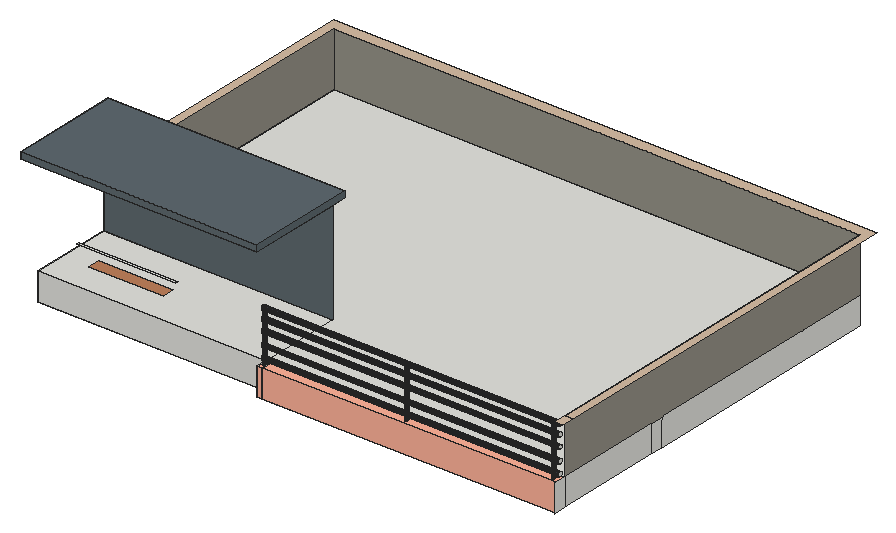
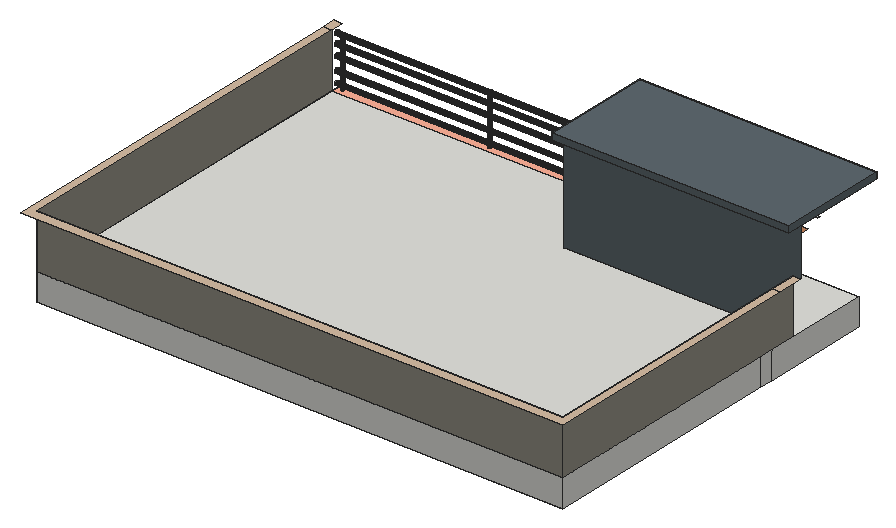
# SketchUp Ruby script. Lengths in inches.
U = 1.inch
M = Sketchup.active_model
def pt(a) = Geom::Point3d.new(a.map { |v| v * U })
def face(e, loops, mat)
  f = e.add_face(loops[0].map { |a| pt(a) })
  loops[1..].each { |l| e.add_face(l.map { |a| pt(a) }).erase! }
  f.material = f.back_material = mat if mat
  f
end
# faces: each face lists its corners as indices into pts; further lists are holes
def faces(e, pts, list, mat = nil) = list.each { |f| face(e, (f[0].is_a?(Array) ? f : [f]).map { |l| l.map { |i| pts[i] } }, mat) }
# xy, xz, yz: faces in a plane at the given z, y or x. An outline is a flat list of corners, or four numbers for a rectangle; further outlines are holes
def ring(l) = l.size == 4 ? [[l[0], l[1]], [l[2], l[1]], [l[2], l[3]], [l[0], l[3]]] : l.each_slice(2).to_a
def flat(e, list, mat, &to3) = list.each { |f| face(e, (f[0].is_a?(Array) ? f : [f]).map { |l| ring(l).map { |u, v| to3.(u, v) } }, mat) }
def xy(e, z, list, mat = nil) = flat(e, list, mat) { |x, y| [x, y, z] }
def xz(e, y, list, mat = nil) = flat(e, list, mat) { |x, z| [x, y, z] }
def yz(e, x, list, mat = nil) = flat(e, list, mat) { |y, z| [x, y, z] }
def lines(e, pts, list) = list.each { |a, b| e.add_line(pt(pts[a]), pt(pts[b])) }
# prism: a flat outline (further loops are holes) pulled along v
def prism(e, loops, v, mat = nil)
  f = face(e, loops, mat); d = Geom::Vector3d.new(v.map { |x| x * U })
  f.pushpull(f.normal.samedirection?(d) ? d.length : -d.length)
end
def box(e, o, s, mat = nil) = prism(e, [[o, [o[0] + s[0], o[1], o[2]], [o[0] + s[0], o[1] + s[1], o[2]], [o[0], o[1] + s[1], o[2]]]], [0, 0, s[2]], mat)
def at(x, y, z, deg = 0) = Geom::Transformation.translation(pt([x, y, z])) * Geom::Transformation.rotation(ORIGIN, Z_AXIS, deg.degrees)
def axes(o, x, y, z) = Geom::Transformation.new([*x, 0, *y, 0, *z, 0, *pt(o).to_a, 1])
def part(name) = M.definitions.add(name)
# library, detail: a bought-in or finely detailed component or shape, given as its bounding box
def library(name, o, s) = part(name).tap { |d| box(d.entities, o, s) }
def detail(e, o, s) = box(e.add_group.entities, o, s)
def put(e, d, t, mat = nil) = e.add_instance(d, t).tap { |i| i.material = mat if mat }
def group(e, t, mat = nil) = e.add_group.tap { |g| g.transformation = t; g.material = mat if mat }.entities
root = M.entities
M.materials.add("[Color B02]").color = [255, 178, 153]
M.materials.add("[Formica Graystone]").color = [149, 146, 135]
M.materials.add("[Formica Laminate Dark]").color = [50, 53, 60]
M.materials.add("[Formica Laminate Light]").color = [213, 189, 164]
M.materials.add("[Formica Speckled Grey]").color = [94, 105, 111]
M.materials.add("[Mirror 02]").color = [229, 229, 229]
M.materials.add("[Translucent Glass Gray]").color = [128, 128, 128]
M.materials["[Translucent Glass Gray]"].alpha = 0.5
M.materials.add("[Wood Veneer 02]").color = [190, 128, 91]
xy(root,233.31,[[241.28,125.15,282.74,137.68]])
xy(root,236.52,[[343.11,125.15,391.96,137.68]])
xy(root,253.98,[[7.28,125.15,478.18,137.68],[7.28,137.68,478.18,359.0625]])
xy(root,253.98,[[211.9,17.0625,211.86,27.5,7.28,27.5,7.28,125.15,478.18,125.15,478.18,28.71,478.21,17.0625,478.18,17.0625,478.17,18.28,216.21,17.09,216.18,27.52,216.17,27.53,216.21,17.09,211.9375,17.0625]],"[Color B02]")
xy(root,278.46,[[216.21,17.09,216.18,27.52,216.17,27.52],[214.34,20.96,214.03,21.01,213.73,21.16,213.48,21.4,213.29,21.71,213.17,22.07,213.13,22.46,213.17,22.85,213.29,23.21,213.48,23.52,213.73,23.76,214.03,23.91,214.34,23.96,214.66,23.91,214.95,23.76,215.2,23.52,215.39,23.21,215.51,22.85,215.55,22.46,215.51,22.07,215.39,21.71,215.2,21.4,214.95,21.16,214.66,21.01],[341.47,20.96,341.16,21.01,340.86,21.16,340.61,21.4,340.42,21.71,340.3,22.07,340.26,22.46,340.3,22.85,340.42,23.21,340.61,23.52,340.86,23.76,341.16,23.91,341.47,23.96,341.79,23.91,342.08,23.76,342.33,23.52,342.52,23.21,342.64,22.85,342.68,22.46,342.64,22.07,342.52,21.71,342.33,21.4,342.08,21.16,341.79,21.01],[473.1,20.96,472.79,21.01,472.49,21.16,472.24,21.4,472.05,21.71,471.93,22.07,471.89,22.46,471.93,22.85,472.05,23.21,472.24,23.52,472.49,23.76,472.79,23.91,473.1,23.96,473.42,23.91,473.71,23.76,473.96,23.52,474.15,23.21,474.27,22.85,474.32,22.46,474.27,22.07,474.15,21.71,473.96,21.4,473.71,21.16,473.42,21.01],[211.9,27.5,216.17,27.52,216.17,27.53,216.18,27.52,478.18,28.71,478.18,359.0625,7.28,359.0625,7.28,101.5625,211.9,101.5625],
  [7.28,27.5,211.9,101.5625],[216.17,27.52,216.18,27.52,216.17,27.53]])
xy(root,278.46,[[[211.9,17.0625,211.9375,17.0625,216.21,17.09,216.17,27.52,211.9,27.5,211.86,27.5],[214.34,20.96,214.03,21.01,213.73,21.16,213.48,21.4,213.29,21.71,213.17,22.07,213.13,22.46,213.17,22.85,213.29,23.21,213.48,23.52,213.73,23.76,214.03,23.91,214.34,23.96,214.66,23.91,214.95,23.76,215.2,23.52,215.39,23.21,215.51,22.85,215.55,22.46,215.51,22.07,215.39,21.71,215.2,21.4,214.95,21.16,214.66,21.01]],[[478.18,17.0625,478.21,17.0625,478.18,28.71,216.18,27.52,216.21,17.09,478.17,18.28],[473.1,20.96,472.79,21.01,472.49,21.16,472.24,21.4,472.05,21.71,471.93,22.07,471.89,22.46,471.93,22.85,472.05,23.21,472.24,23.52,472.49,23.76,472.79,23.91,473.1,23.96,473.42,23.91,473.71,23.76,473.96,23.52,474.15,23.21,474.27,22.85,474.32,22.46,474.27,22.07,474.15,21.71,473.96,21.4,473.71,21.16,473.42,21.01],[341.47,20.96,341.16,21.01,340.86,21.16,340.61,21.4,340.42,21.71,340.3,22.07,340.26,22.46,340.3,22.85,340.42,23.21,340.61,23.52,340.86,23.76,341.16,23.91,341.47,23.96,341.79,23.91,342.08,23.76,342.33,23.52,342.52,23.21,342.64,22.85,342.68,22.46,342.64,22.07,342.52,21.71,342.33,21.4,342.08,21.16,341.79,21.01]]],"[Color B02]")
xy(root,306.94,[[63.47,14.6875,129.94,25.8125]],"[Wood Veneer 02]")
xy(root,321.27,[[52.1,14.6875,141.31,17.0625]])
xy(root,323.28,[[473.1,20.96,473.42,21.01,473.71,21.16,473.96,21.4,474.15,21.71,474.27,22.07,474.32,22.46,474.27,22.85,474.15,23.21,473.96,23.52,473.71,23.76,473.42,23.91,473.1,23.96,472.79,23.91,472.49,23.76,472.24,23.52,472.05,23.21,471.93,22.85,471.89,22.46,471.93,22.07,472.05,21.71,472.24,21.4,472.49,21.16,472.79,21.01]])
xy(root,323.89,[[341.47,20.96,341.79,21.01,342.08,21.16,342.33,21.4,342.52,21.71,342.64,22.07,342.66,22.1875,340.29,22.1875,340.3,22.07,340.42,21.71,340.61,21.4,340.86,21.16,341.16,21.01],[340.29,22.1875,342.66,22.1875,342.68,22.46,342.64,22.85,342.52,23.21,342.33,23.52,342.08,23.76,341.79,23.91,341.47,23.96,341.16,23.91,340.86,23.76,340.61,23.52,340.42,23.21,340.3,22.85,340.26,22.46]])
xy(root,324.26,[[214.34,20.96,214.66,21.01,214.95,21.16,215.2,21.4,215.39,21.71,215.51,22.07,215.55,22.46,215.55,22.47,213.13,22.47,213.13,22.46,213.17,22.07,213.29,21.71,213.48,21.4,213.73,21.16,214.03,21.01],[213.13,22.47,215.55,22.47,215.51,22.85,215.39,23.21,215.2,23.52,214.95,23.76,214.66,23.91,214.34,23.96,214.03,23.91,213.73,23.76,213.48,23.52,213.29,23.21,213.17,22.85]])
xy(root,327.42,[[478.18,17.0625,485.46,28.71],[478.18,28.71,485.46,28.71,485.46,368.0625,0,368.0625,0,125.15,7.28,125.15,7.28,359.0625,478.18,359.0625],[0,101.5625,7.28,125.15]],"[Formica Laminate Light]")
xy(root,370.36,[[0,17.0625,211.9,101.5625],[0,101.5625,211.9,115.3125]])
xy(root,376.1875,[[0,17.0625,211.9,115.3125]],"[Formica Speckled Grey]")
xz(root,17.0625,[[211.9,253.98,211.9375,278.46],[478.18,253.98,478.21,278.46]])
xz(root,17.0625,[[0,370.36,211.9,376.1875]],"[Formica Speckled Grey]")
xz(root,27.5,[[7.28,253.98,211.86,278.46],[211.86,253.98,211.9,278.46]])
xz(root,101.5625,[[7.28,278.46,7.28,327.42,0,327.42,0,370.36,211.9,370.36,211.9,278.46]],"[Formica Speckled Grey]")
xz(root,115.3125,[[0,370.36,211.9,376.1875]],"[Formica Speckled Grey]")
xz(root,125.15,[[245.46,221.85,260.12,228.03],[263.78,221.85,278.56,228.03]],"[Mirror 02]")
xz(root,125.15,[[346.84,218.58,365.15,225.02],[369.6875,218.58,388.23,225.02],[346.84,225.02,365.15,231.81],[369.6875,225.02,388.23,231.81]],"[Translucent Glass Gray]")
xz(root,359.0625,[[7.28,253.98,478.18,278.46]])
xz(root,359.0625,[[7.28,278.46,478.18,327.42]],"[Formica Graystone]")
yz(root,0,[[17.0625,370.36,115.3125,376.1875]],"[Formica Speckled Grey]")
yz(root,7.28,[[27.5,253.98,125.15,278.46],[125.15,253.98,137.68,278.46],[137.68,253.98,359.0625,278.46]])
yz(root,7.28,[[101.5625,278.46,359.0625,327.42]],"[Formica Graystone]")
yz(root,211.9,[[17.0625,370.36,115.3125,376.1875]],"[Formica Speckled Grey]")
yz(root,478.18,[[28.71,253.98,125.15,278.46],[125.15,253.98,137.68,278.46],[137.68,253.98,359.0625,278.46],[23.7,280.86,24.16,280.92,24.58,281.1,24.94,281.38,25.22,281.75,25.4,282.18,25.45,282.64,25.4,283.11,25.22,283.54,24.94,283.91,24.58,284.19,24.16,284.37,23.7,284.43,23.25,284.37,22.83,284.19,22.47,283.91,22.1875,283.54,22.01,283.11,21.95,282.64,22.01,282.18,22.1875,281.75,22.47,281.38,22.83,281.1,23.25,280.92],[23.7,291,24.16,291.06,24.58,291.23,24.94,291.52,25.22,291.89,25.4,292.32,25.45,292.78,25.4,293.24,25.22,293.67,24.94,294.04,24.58,294.33,24.16,294.5,23.7,294.57,23.25,294.5,22.83,294.33,22.47,294.04,22.1875,293.67,22.01,293.24,21.95,292.78,22.01,292.32,22.1875,291.89,22.47,291.52,22.83,291.23,23.25,291.06],
  [23.7,302.73,24.16,302.79,24.58,302.96,24.94,303.25,25.22,303.62,25.4,304.05,25.45,304.51,25.4,304.97,25.22,305.4,24.94,305.77,24.58,306.06,24.16,306.23,23.7,306.3,23.25,306.23,22.83,306.06,22.47,305.77,22.1875,305.4,22.01,304.97,21.95,304.51,22.01,304.05,22.1875,303.62,22.47,303.25,22.83,302.96,23.25,302.79],[23.7,312.48,24.16,312.54,24.58,312.72,24.94,313,25.22,313.37,25.4,313.8,25.45,314.26,25.4,314.73,25.22,315.16,24.94,315.53,24.58,315.81,24.16,315.99,23.7,316.05,23.25,315.99,22.83,315.81,22.47,315.53,22.1875,315.16,22.01,314.73,21.95,314.26,22.01,313.8,22.1875,313.37,22.47,313,22.83,312.72,23.25,312.54],[23.7,321.21,24.16,321.27,24.58,321.45,24.94,321.74,25.22,322.11,25.4,322.54,25.45,323,25.4,323.46,25.22,323.89,24.94,324.26,24.58,324.54,24.16,324.72,23.7,324.78,23.25,324.72,22.83,324.54,22.47,324.26,22.1875,323.89,22.01,323.46,21.95,323,22.01,322.54,22.1875,322.11,22.47,321.74,22.83,321.45,23.25,321.27]])
yz(root,478.18,[[28.71,278.46,359.0625,327.42]],"[Formica Graystone]")
p = [[211.9375,17.0625,253.98],[216.21,17.09,253.98],[216.21,17.09,278.46],[211.9375,17.0625,278.46],[211.86,27.5,278.46],[211.86,27.5,253.98],
  [211.9,17.0625,253.98],[211.9,17.0625,278.46],[216.18,27.52,253.98],[216.18,27.52,278.46],[478.17,18.28,253.98],[478.17,18.28,278.46],
  [216.17,27.53,253.98],[216.17,27.53,278.46],[216.17,27.52,278.46],[478.18,28.71,253.98],[478.18,28.71,278.46],[478.21,17.0625,278.46],
  [478.21,17.0625,253.98],[478.18,17.0625,253.98],[478.18,17.0625,278.46],[213.73,21.16,278.46],[214.03,21.01,278.46],[214.03,21.01,324.26],
  [213.73,21.16,324.26],[214.34,20.96,278.46],[214.34,20.96,324.26],[214.66,21.01,278.46],[214.66,21.01,324.26],[214.95,21.16,278.46],
  [214.95,21.16,324.26],[340.86,21.16,278.46],[341.16,21.01,278.46],[341.16,21.01,323.89],[340.86,21.16,323.89],[341.47,20.96,278.46],
  [341.47,20.96,323.89],[341.79,21.01,278.46],[341.79,21.01,323.89],[342.08,21.16,278.46],[342.08,21.16,323.89],[472.49,21.16,278.46],
  [472.79,21.01,278.46],[472.79,21.01,323.28],[472.49,21.16,323.28],[473.1,20.96,278.46],[473.1,20.96,323.28],[473.42,21.01,278.46],
  [473.42,21.01,323.28],[473.71,21.16,278.46],[473.71,21.16,323.28],[213.48,21.4,278.46],[213.48,21.4,324.26],[215.2,21.4,278.46],
  [215.2,21.4,324.26],[340.61,21.4,278.46],[340.61,21.4,323.89],[342.33,21.4,278.46],[342.33,21.4,323.89],[472.24,21.4,278.46],
  [472.24,21.4,323.28],[473.96,21.4,278.46],[473.96,21.4,323.28],[213.29,21.71,278.46],[213.29,21.71,324.26],[215.39,21.71,278.46],
  [215.39,21.71,324.26],[340.42,21.71,278.46],[340.42,21.71,323.89],[342.52,21.71,278.46],[342.52,21.71,323.89],[472.05,21.71,278.46],
  [472.05,21.71,323.28],[474.15,21.71,278.46],[474.15,21.71,323.28],[213.17,22.07,278.46],[213.17,22.07,324.26],[215.51,22.07,278.46],
  [215.51,22.07,324.26],[340.3,22.07,278.46],[340.3,22.07,323.89],[342.64,22.07,278.46],[342.64,22.07,323.89],[471.93,22.07,278.46],
  [471.93,22.07,323.28],[474.27,22.07,278.46],[474.27,22.07,323.28],[213.13,22.46,278.46],[213.13,22.46,324.26],[215.55,22.46,278.46],
  [215.55,22.46,324.26],[340.26,22.46,278.46],[340.29,22.1875,323.89],[340.26,22.46,323.89],[342.68,22.46,278.46],[342.68,22.46,323.89],
  [342.66,22.1875,323.89],[471.89,22.46,278.46],[471.89,22.46,323.28],[474.32,22.46,278.46],[474.32,22.46,323.28],[213.17,22.85,278.46],
  [213.13,22.47,324.26],[213.17,22.85,324.26],[215.51,22.85,278.46],[215.51,22.85,324.26],[215.55,22.47,324.26],[340.3,22.85,278.46],
  [340.3,22.85,323.89],[342.64,22.85,278.46],[342.64,22.85,323.89],[471.93,22.85,278.46],[471.93,22.85,323.28],[474.27,22.85,278.46],
  [474.27,22.85,323.28],[213.29,23.21,278.46],[213.29,23.21,324.26],[215.39,23.21,278.46],[215.39,23.21,324.26],[340.42,23.21,278.46],
  [340.42,23.21,323.89],[342.52,23.21,278.46],[342.52,23.21,323.89],[472.05,23.21,278.46],[472.05,23.21,323.28],[474.15,23.21,278.46],
  [474.15,23.21,323.28],[213.48,23.52,278.46],[213.48,23.52,324.26],[215.2,23.52,278.46],[215.2,23.52,324.26],[340.61,23.52,278.46],
  [340.61,23.52,323.89],[342.33,23.52,278.46],[342.33,23.52,323.89],[472.24,23.52,278.46],[472.24,23.52,323.28],[473.96,23.52,278.46],
  [473.96,23.52,323.28],[213.73,23.76,278.46],[213.73,23.76,324.26],[214.95,23.76,278.46],[214.95,23.76,324.26],[340.86,23.76,278.46],
  [340.86,23.76,323.89],[342.08,23.76,278.46],[342.08,23.76,323.89],[472.49,23.76,278.46],[472.49,23.76,323.28],[473.71,23.76,278.46],
  [473.71,23.76,323.28],[214.03,23.91,278.46],[214.03,23.91,324.26],[214.66,23.91,278.46],[214.66,23.91,324.26],[341.16,23.91,278.46],
  [341.16,23.91,323.89],[341.79,23.91,278.46],[341.79,23.91,323.89],[472.79,23.91,278.46],[472.79,23.91,323.28],[473.42,23.91,278.46],
  [473.42,23.91,323.28],[214.34,23.96,278.46],[214.34,23.96,324.26],[341.47,23.96,278.46],[341.47,23.96,323.89],[473.1,23.96,278.46],
  [473.1,23.96,323.28],[478.18,23.25,280.92],[478.18,22.83,281.1],[211.9,22.83,281.1],[211.9,23.25,280.92],[478.18,23.7,280.86],
  [211.9,23.7,280.86],[478.18,24.16,280.92],[211.9,24.16,280.92],[478.18,24.58,281.1],[211.9,24.58,281.1],[478.18,22.47,281.38],
  [211.9,22.47,281.38],[478.18,24.94,281.38],[211.9,24.94,281.38],[478.18,22.1875,281.75],[211.9,22.1875,281.75],[478.18,25.22,281.75],
  [211.9,25.22,281.75],[478.18,22.01,282.18],[211.9,22.01,282.18],[478.18,25.4,282.18],[211.9,25.4,282.18],[478.18,21.95,282.64],
  [211.9,21.95,282.64],[478.18,25.45,282.64],[211.9,25.45,282.64],[478.18,22.01,283.11],[211.9,22.01,283.11],[478.18,25.4,283.11],
  [211.9,25.4,283.11],[478.18,22.1875,283.54],[211.9,22.1875,283.54],[478.18,25.22,283.54],[211.9,25.22,283.54],[478.18,22.47,283.91],
  [211.9,22.47,283.91],[478.18,24.94,283.91],[211.9,24.94,283.91],[478.18,22.83,284.19],[211.9,22.83,284.19],[478.18,24.58,284.19],
  [211.9,24.58,284.19],[478.18,23.25,284.37],[211.9,23.25,284.37],[478.18,24.16,284.37],[211.9,24.16,284.37],[478.18,23.7,284.43],
  [211.9,23.7,284.43],[478.18,23.7,291],[478.18,23.25,291.06],[211.9,23.25,291.06],[211.9,23.7,291],[478.18,24.16,291.06],
  [211.9,24.16,291.06],[478.18,22.83,291.23],[211.9,22.83,291.23],[478.18,24.58,291.23],[211.9,24.58,291.23],[478.18,22.47,291.52],
  [211.9,22.47,291.52],[478.18,24.94,291.52],[211.9,24.94,291.52],[478.18,22.1875,291.89],[211.9,22.1875,291.89],[478.18,25.22,291.89],
  [211.9,25.22,291.89],[478.18,22.01,292.32],[211.9,22.01,292.32],[478.18,25.4,292.32],[211.9,25.4,292.32],[478.18,21.95,292.78],
  [211.9,21.95,292.78],[478.18,25.45,292.78],[211.9,25.45,292.78],[478.18,22.01,293.24],[211.9,22.01,293.24],[478.18,25.4,293.24],
  [211.9,25.4,293.24],[478.18,22.1875,293.67],[211.9,22.1875,293.67],[478.18,25.22,293.67],[211.9,25.22,293.67],[478.18,22.47,294.04],
  [211.9,22.47,294.04],[478.18,24.94,294.04],[211.9,24.94,294.04],[478.18,22.83,294.33],[211.9,22.83,294.33],[478.18,24.58,294.33],
  [211.9,24.58,294.33],[478.18,23.25,294.5],[211.9,23.25,294.5],[478.18,24.16,294.5],[211.9,24.16,294.5],[478.18,23.7,294.57],
  [211.9,23.7,294.57],[478.18,23.7,302.73],[478.18,23.25,302.79],[211.9,23.25,302.79],[211.9,23.7,302.73],[478.18,24.16,302.79],
  [211.9,24.16,302.79],[478.18,22.83,302.96],[211.9,22.83,302.96],[478.18,24.58,302.96],[211.9,24.58,302.96],[478.18,22.47,303.25],
  [211.9,22.47,303.25],[478.18,24.94,303.25],[211.9,24.94,303.25],[478.18,22.1875,303.62],[211.9,22.1875,303.62],[478.18,25.22,303.62],
  [211.9,25.22,303.62],[478.18,22.01,304.05],[211.9,22.01,304.05],[478.18,25.4,304.05],[211.9,25.4,304.05],[478.18,21.95,304.51],
  [211.9,21.95,304.51],[478.18,25.45,304.51],[211.9,25.45,304.51],[478.18,22.01,304.97],[211.9,22.01,304.97],[478.18,25.4,304.97],
  [211.9,25.4,304.97],[478.18,22.1875,305.4],[211.9,22.1875,305.4],[478.18,25.22,305.4],[211.9,25.22,305.4],[478.18,22.47,305.77],
  [211.9,22.47,305.77],[478.18,24.94,305.77],[211.9,24.94,305.77],[478.18,22.83,306.06],[211.9,22.83,306.06],[478.18,24.58,306.06],
  [211.9,24.58,306.06],[478.18,23.25,306.23],[211.9,23.25,306.23],[478.18,24.16,306.23],[211.9,24.16,306.23],[478.18,23.7,306.3],
  [211.9,23.7,306.3],[478.18,23.25,312.54],[478.18,22.83,312.72],[211.9,22.83,312.72],[211.9,23.25,312.54],[478.18,23.7,312.48],
  [211.9,23.7,312.48],[478.18,24.16,312.54],[211.9,24.16,312.54],[478.18,24.58,312.72],[211.9,24.58,312.72],[478.18,22.47,313],
  [211.9,22.47,313],[478.18,24.94,313],[211.9,24.94,313],[478.18,22.1875,313.37],[211.9,22.1875,313.37],[478.18,25.22,313.37],
  [211.9,25.22,313.37],[478.18,22.01,313.8],[211.9,22.01,313.8],[478.18,25.4,313.8],[211.9,25.4,313.8],[478.18,21.95,314.26],
  [211.9,21.95,314.26],[478.18,25.45,314.26],[211.9,25.45,314.26],[478.18,22.01,314.73],[211.9,22.01,314.73],[478.18,25.4,314.73],
  [211.9,25.4,314.73],[478.18,22.1875,315.16],[211.9,22.1875,315.16],[478.18,25.22,315.16],[211.9,25.22,315.16],[478.18,22.47,315.53],
  [211.9,22.47,315.53],[478.18,24.94,315.53],[211.9,24.94,315.53],[478.18,22.83,315.81],[211.9,22.83,315.81],[478.18,24.58,315.81],
  [211.9,24.58,315.81],[478.18,23.25,315.99],[211.9,23.25,315.99],[478.18,24.16,315.99],[211.9,24.16,315.99],[478.18,23.7,316.05],
  [211.9,23.7,316.05],[478.18,23.7,321.21],[478.18,23.25,321.27],[211.9,23.25,321.27],[211.9,23.7,321.21],[478.18,24.16,321.27],
  [211.9,24.16,321.27],[478.18,22.83,321.45],[211.9,22.83,321.45],[478.18,24.58,321.45],[211.9,24.58,321.45],[478.18,22.47,321.74],
  [211.9,22.47,321.74],[478.18,24.94,321.74],[211.9,24.94,321.74],[478.18,22.1875,322.11],[211.9,22.1875,322.11],[478.18,25.22,322.11],
  [211.9,25.22,322.11],[478.18,22.01,322.54],[211.9,22.01,322.54],[478.18,25.4,322.54],[211.9,25.4,322.54],[478.18,21.95,323],
  [211.9,21.95,323],[478.18,25.45,323],[211.9,25.45,323],[478.18,22.01,323.46],[211.9,22.01,323.46],[478.18,25.4,323.46],
  [211.9,25.4,323.46],[478.18,22.1875,323.89],[211.9,22.1875,323.89],[478.18,25.22,323.89],[211.9,25.22,323.89],[478.18,22.47,324.26],
  [211.9,22.47,324.26],[478.18,24.94,324.26],[211.9,24.94,324.26],[478.18,22.83,324.54],[211.9,22.83,324.54],[478.18,24.58,324.54],
  [211.9,24.58,324.54],[478.18,23.25,324.72],[211.9,23.25,324.72],[478.18,24.16,324.72],[211.9,24.16,324.72],[478.18,23.7,324.78],
  [211.9,23.7,324.78]]
faces(root,p,[[0,1,2,3],[1,10,11,2]],"[Color B02]")
faces(root,p,[[4,5,6,7],[8,1,2,9],[12,13,14,2,1],[15,16,17,18],[19,20,11,10],[12,8,9,13]])
faces(root,p,[[21,22,23,24],[22,25,26,23],[25,27,28,26],[27,29,30,28],[31,32,33,34],[32,35,36,33],[35,37,38,36],[37,39,40,38],
  [41,42,43,44],[42,45,46,43],[45,47,48,46],[47,49,50,48],[51,21,24,52],[29,53,54,30],[55,31,34,56],[39,57,58,40],
  [59,41,44,60],[49,61,62,50],[63,51,52,64],[53,65,66,54],[67,55,56,68],[57,69,70,58],[71,59,60,72],[61,73,74,62],
  [75,63,64,76],[65,77,78,66],[79,67,68,80],[69,81,82,70],[83,71,72,84],[73,85,86,74],[87,75,76,88],[77,89,90,78],
  [91,79,80,92,93],[81,94,95,96,82],[97,83,84,98],[85,99,100,86],[101,87,88,102,103],[89,104,105,106,90],[107,91,93,108],[94,109,110,95],
  [111,97,98,112],[99,113,114,100],[115,101,103,116],[104,117,118,105],[119,107,108,120],[109,121,122,110],[123,111,112,124],[113,125,126,114],
  [127,115,116,128],[117,129,130,118],[131,119,120,132],[121,133,134,122],[135,123,124,136],[125,137,138,126],[139,127,128,140],[129,141,142,130],
  [143,131,132,144],[133,145,146,134],[147,135,136,148],[137,149,150,138],[151,139,140,152],[141,153,154,142],[155,143,144,156],[145,157,158,146],
  [159,147,148,160],[149,161,162,150],[163,151,152,164],[153,163,164,154],[165,155,156,166],[157,165,166,158],[167,159,160,168],[161,167,168,162],
  [169,170,171,172],[173,169,172,174],[175,173,174,176],[177,175,176,178],[170,179,180,171],[181,177,178,182],[179,183,184,180],[185,181,182,186],
  [183,187,188,184],[189,185,186,190],[187,191,192,188],[193,189,190,194],[191,195,196,192],[197,193,194,198],[195,199,200,196],[201,197,198,202],
  [199,203,204,200],[205,201,202,206],[203,207,208,204],[209,205,206,210],[207,211,212,208],[213,209,210,214],[211,215,216,212],[215,213,214,216],
  [217,218,219,220],[221,217,220,222],[218,223,224,219],[225,221,222,226],[223,227,228,224],[229,225,226,230],[227,231,232,228],[233,229,230,234],
  [231,235,236,232],[237,233,234,238],[235,239,240,236],[241,237,238,242],[239,243,244,240],[245,241,242,246],[243,247,248,244],[249,245,246,250],
  [247,251,252,248],[253,249,250,254],[251,255,256,252],[257,253,254,258],[255,259,260,256],[261,257,258,262],[259,263,264,260],[263,261,262,264],
  [265,266,267,268],[269,265,268,270],[266,271,272,267],[273,269,270,274],[271,275,276,272],[277,273,274,278],[275,279,280,276],[281,277,278,282],
  [279,283,284,280],[285,281,282,286],[283,287,288,284],[289,285,286,290],[287,291,292,288],[293,289,290,294],[291,295,296,292],[297,293,294,298],
  [295,299,300,296],[301,297,298,302],[299,303,304,300],[305,301,302,306],[303,307,308,304],[309,305,306,310],[307,311,312,308],[311,309,310,312],
  [313,314,315,316],[317,313,316,318],[319,317,318,320],[321,319,320,322],[314,323,324,315],[325,321,322,326],[323,327,328,324],[329,325,326,330],
  [327,331,332,328],[333,329,330,334],[331,335,336,332],[337,333,334,338],[335,339,340,336],[341,337,338,342],[339,343,344,340],[345,341,342,346],
  [343,347,348,344],[349,345,346,350],[347,351,352,348],[353,349,350,354],[351,355,356,352],[357,353,354,358],[355,359,360,356],[359,357,358,360],
  [361,362,363,364],[365,361,364,366],[362,367,368,363],[369,365,366,370],[367,371,372,368],[373,369,370,374],[371,375,376,372],[377,373,374,378],
  [375,379,380,376],[381,377,378,382],[379,383,384,380],[385,381,382,386],[383,387,388,384],[389,385,386,390],[387,391,96,92,392,388],[393,389,390,394],
  [391,395,106,102,396,392,92,96],[397,393,394,398],[395,399,400,396,102,106],[401,397,398,402],[399,403,404,400],[405,401,402,406],[403,407,408,404],[407,405,406,408]],"[Formica Laminate Dark]")
